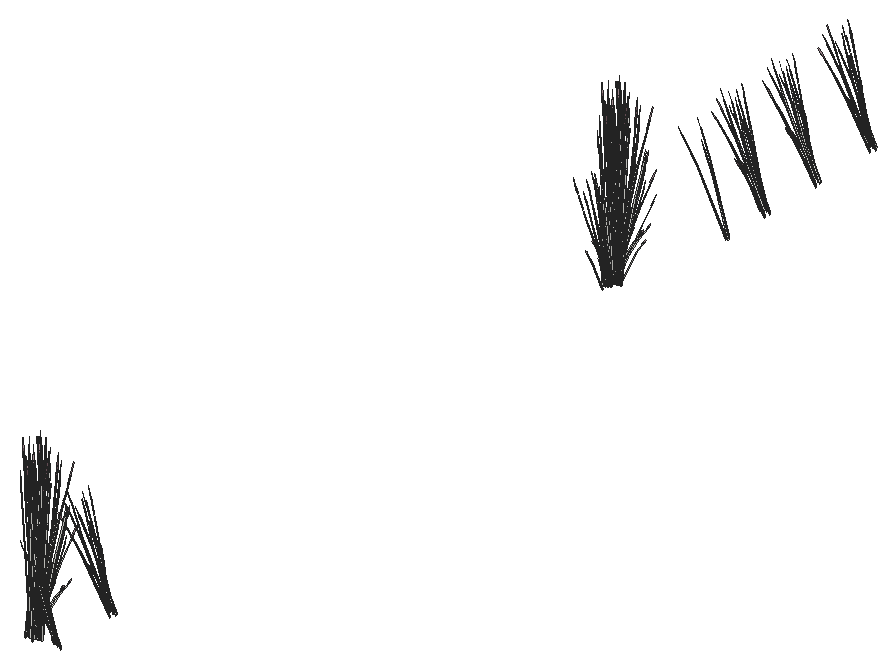
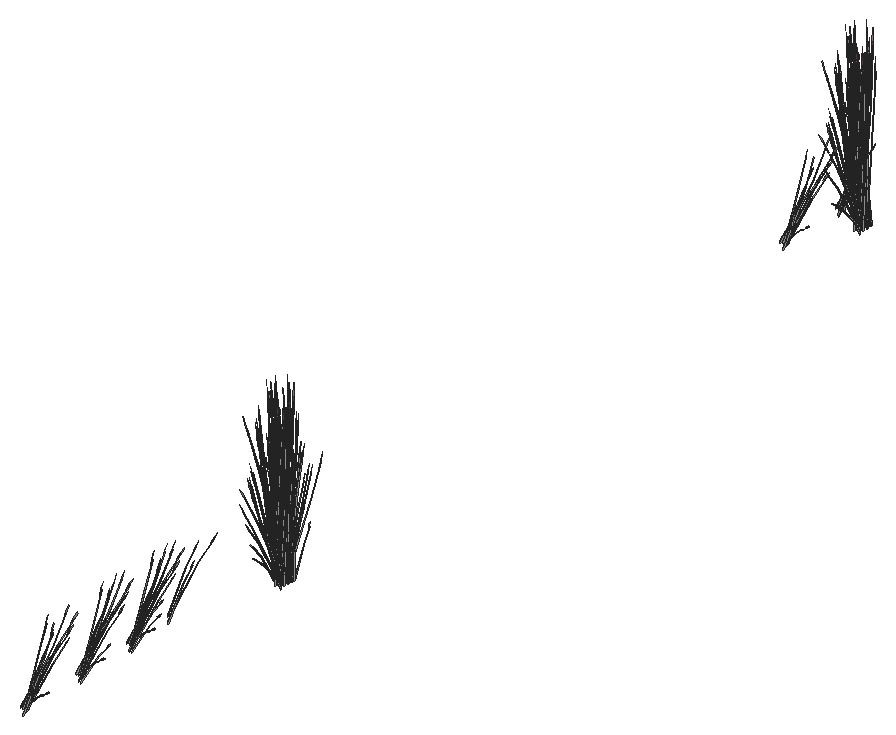
# SketchUp Ruby script. Lengths in inches.
U = 1.inch
M = Sketchup.active_model
def pt(a) = Geom::Point3d.new(a.map { |v| v * U })
def face(e, loops, mat)
  f = e.add_face(loops[0].map { |a| pt(a) })
  loops[1..].each { |l| e.add_face(l.map { |a| pt(a) }).erase! }
  f.material = f.back_material = mat if mat
  f
end
# faces: each face lists its corners as indices into pts; further lists are holes
def faces(e, pts, list, mat = nil) = list.each { |f| face(e, (f[0].is_a?(Array) ? f : [f]).map { |l| l.map { |i| pts[i] } }, mat) }
# xy, xz, yz: faces in a plane at the given z, y or x. An outline is a flat list of corners, or four numbers for a rectangle; further outlines are holes
def ring(l) = l.size == 4 ? [[l[0], l[1]], [l[2], l[1]], [l[2], l[3]], [l[0], l[3]]] : l.each_slice(2).to_a
def flat(e, list, mat, &to3) = list.each { |f| face(e, (f[0].is_a?(Array) ? f : [f]).map { |l| ring(l).map { |u, v| to3.(u, v) } }, mat) }
def xy(e, z, list, mat = nil) = flat(e, list, mat) { |x, y| [x, y, z] }
def xz(e, y, list, mat = nil) = flat(e, list, mat) { |x, z| [x, y, z] }
def yz(e, x, list, mat = nil) = flat(e, list, mat) { |y, z| [x, y, z] }
def lines(e, pts, list) = list.each { |a, b| e.add_line(pt(pts[a]), pt(pts[b])) }
# prism: a flat outline (further loops are holes) pulled along v
def prism(e, loops, v, mat = nil)
  f = face(e, loops, mat); d = Geom::Vector3d.new(v.map { |x| x * U })
  f.pushpull(f.normal.samedirection?(d) ? d.length : -d.length)
end
def box(e, o, s, mat = nil) = prism(e, [[o, [o[0] + s[0], o[1], o[2]], [o[0] + s[0], o[1] + s[1], o[2]], [o[0], o[1] + s[1], o[2]]]], [0, 0, s[2]], mat)
def at(x, y, z, deg = 0) = Geom::Transformation.translation(pt([x, y, z])) * Geom::Transformation.rotation(ORIGIN, Z_AXIS, deg.degrees)
def axes(o, x, y, z) = Geom::Transformation.new([*x, 0, *y, 0, *z, 0, *pt(o).to_a, 1])
def part(name) = M.definitions.add(name)
# library, detail: a bought-in or finely detailed component or shape, given as its bounding box
def library(name, o, s) = part(name).tap { |d| box(d.entities, o, s) }
def detail(e, o, s) = box(e.add_group.entities, o, s)
def put(e, d, t, mat = nil) = e.add_instance(d, t).tap { |i| i.material = mat if mat }
def group(e, t, mat = nil) = e.add_group.tap { |g| g.transformation = t; g.material = mat if mat }.entities
root = M.entities
M.materials.add("LightPink_Translucent").color = [144, 107, 117]
M.materials["LightPink_Translucent"].alpha = 0.75
c1 = part("blade")
p = [[2.15,0.21,22],[0,0.17,0],[0.09,0.45,0],[2.18,0.31,22],[2.29,0.31,22],[0.38,0.45,0],
  [2.48,0.24,33],[2.49,0.24,33],[2.48,0.22,33]]
faces(c1.entities,p,[[0,1,2,3],[4,5,2,3],[6,3,4,7],[8,0,3,6]])
c2 = part("seeds")
p = [[0.3,-0.1,1.38],[-0.01,-0.03,1.59],[-0.01,-0.03,0.03],[0.14,-0.07,-0.07],[0.29,-0.03,3],[0.15,0.01,3.11]]
faces(c2.entities,p,[[0,1,2,3],[1,0,4,5]],"LightPink_Translucent")
c3 = part("blade with seeds")
put(c3.entities,c1,at(0,0,0))
put(c3.entities,c2,axes([2.4,0.25,30.99],[1.5799,-0.05474,1.17369],[-0.12525,1.92788,0.29478],[-0.07173,-0.02425,1.56792]))
put(root,c3,axes([492.53,187.29,1.91],[-0.82508,0.03772,0.44739],[-0.07462,-0.62614,-0.21531],[0.14771,-0.06346,1.43643]))
put(root,c3,axes([492.5,187.51,1.55],[0.33034,0.68327,0.45755],[-0.94388,0.2376,0.17955],[0.01154,-0.12555,1.58856]))
put(root,c3,axes([502.6,185.86,3.72],[-0.63144,-0.17046,-0.35414],[0.18417,-0.49731,0.4572],[-0.25423,0.0456,0.87481]))
put(root,c3,axes([492.33,188.05,1.91],[-0.36864,0.55059,0.44739],[-0.76598,-0.26498,-0.21531],[0,-0.12692,1.43643]))
put(root,c3,axes([493.6875,187.57,1.4],[0,-0.70701,0],[0.95008,0,0],[0,0,1.79456]))
put(root,c3,axes([494.84,185.9375,1.67],[-0.7111,-0.30552,0.49651],[0.42504,-0.54784,0],[0.16196,0.06958,1.57504]))
put(root,c3,axes([493.24,187.125,1.55],[-0.62999,0.55453,0.45755],[-0.74845,-0.4895,0.17955],[0.15188,-0.05534,1.58856]))
put(root,c3,axes([493.92,188.12,1.49],[-0.70674,-0.52593,-0.06131],[0.70717,-0.52625,0],[-0.02468,-0.01837,1.75571]))
put(root,c3,axes([492.14,186.21,1.67],[-0.21949,0.60727,0.17642],[-0.8032,-0.17185,0.35086],[0.13875,-0.00296,1.60407]))
put(root,c3,axes([493.82,186.89,1.81],[0.14658,-0.54532,0.1448],[0.71613,0.09466,-0.41347],[0.13033,0.05599,1.26744]))
put(root,c3,axes([504.52,185.78,2.53],[0.21597,-0.08839,1.77064],[0.07448,0.61717,0.13857],[-0.4678,0.08189,0.63284]))
put(root,c3,axes([493.51,187.03,1.91],[-0.45644,-0.51287,0.44739],[0.69137,-0.36116,-0.21531],[0.14771,0.06346,1.43643]))
put(root,c3,axes([492.07,189.34,1.67],[0.81646,-0.16218,0.17642],[0.20161,0.60355,0.35086],[-0.07282,-0.08794,1.60407]))
put(root,c3,axes([502.2,186.1875,3.91],[-0.12407,0.07933,1.74944],[0.01055,0.57963,-0.27667],[-0.2844,0.07538,0.14031]))
put(root,c3,axes([503.03,186.11,3.875],[-0.20584,0.55581,-0.51099],[-0.70573,-0.19051,-0.3958],[-0.28414,0.05097,0.97773]))
put(root,c3,axes([494.33,187.73,1.4],[0.85008,0,0],[0,0.63259,0],[0,0,1.78407]))
put(root,c3,axes([494.57,186.24,1.67],[-0.81646,0.16218,0.17642],[-0.20161,-0.60355,0.35086],[0.07282,0.08794,1.60407]))
put(root,c3,axes([494.06,187.41,1.57],[-0.96033,-0.12874,0.49198],[0.19544,-0.7271,0.19306],[0.14034,0.07021,1.70813]))
put(root,c3,axes([493.29,189.2,1.4],[-0.24791,-0.5268,0],[0.70791,-0.18448,0],[0,0,1.54371]))
put(root,c3,axes([494.22,189.13,1.38],[0.79769,-0.20732,-0.19198],[0.2803,0.59721,0.00008],[0.08805,-0.02292,1.73897]))
put(root,c3,axes([494.49,189.375,1.67],[0.21949,-0.60727,0.17642],[0.8032,0.17185,0.35086],[-0.13875,0.00296,1.60407]))
put(root,c3,axes([494.3125,188,1.41],[0.53038,0.39469,0],[-0.53038,0.39469,0],[0,0,1.69266]))
put(root,c3,axes([495.75,187.83,1.67],[-0.59697,-0.44509,0.17642],[0.60159,-0.4317,0.35086],[-0.06593,0.0909,1.60407]))
put(root,c3,axes([503,186.4,3.07],[0.26363,-0.12925,1.71376],[0.22195,0.59723,0.13857],[-0.41388,0.13498,0.73262]))
put(root,c3,axes([493.12,189.44,1.39],[-0.76598,-0.27433,0],[0.36864,-0.57001,0],[0,0,1.62707]))
put(root,c3,axes([494.31,187.54,1.91],[0.36864,-0.55059,0.44739],[0.76598,0.26498,-0.21531],[0,0.12692,1.43643]))
put(root,c3,axes([494.16,187.85,1.48],[0,0.70667,-0.05637],[-0.95008,0,0],[0,0.02221,1.79368]))
put(root,c3,axes([494.23,187.35,1.4],[0.45644,0.51287,-0.44739],[-0.69137,0.36116,0.21531],[0.14771,0.06346,1.43643]))
put(root,c3,axes([502.18,187.42,1.78],[0.26405,0.05016,1.43002],[0.17019,0.51235,-0.30754],[-0.35868,0.0959,0.61141]))
put(root,c3,axes([500.82,186.78,3.9],[0.09697,0.01639,1.77383],[0.29997,0.53988,-0.16761],[-0.1985,0.1417,0.31391]))
put(root,c3,axes([496.24,187.84,1.67],[0,-0.61104,0.49651],[0.85008,0,0],[0,0.13917,1.57504]))
put(root,c3,axes([494.11,188.3,1.91],[0.82508,-0.03772,0.44739],[0.07462,0.62614,-0.21531],[-0.14771,0.06346,1.43643]))
put(root,c3,axes([494.625,187.66,1.81],[0.70791,-0.1782,0.1448],[0.24791,0.50885,-0.41347],[0,0.11199,1.26744]))
put(root,c3,axes([493.99,189.45,1.4],[0.76598,0.27433,0],[-0.36864,0.57001,0],[0,0,1.74954]))
put(root,c3,axes([494.125,188.57,1.81],[0.56134,0.36712,0.1448],[-0.46823,0.41419,-0.41347],[-0.13033,0.05599,1.26744]))
put(root,c3,axes([494.72,189.7,1.67],[0.7111,-0.30552,0.49651],[0.42504,0.54784,0],[-0.16196,0.06958,1.57504]))
put(root,c3,axes([493.71,189.22,1.48],[0.33034,0.70197,-0.06012],[-0.94388,0.24598,0],[0.01154,0.02451,1.72173]))
put(root,c3,axes([496.4375,188.3,1.39],[-0.94962,-0.00489,-0.04976],[0,-0.68292,0.49943],[-0.02984,0.15546,1.58352]))
put(root,c3,axes([494.38,187.7,1.86],[0.85568,0.29155,-0.29095],[-0.41201,0.61537,-0.50002],[0.02689,0.15109,1.59708]))
put(root,c3,axes([496.24,188.4,1.22],[-0.53038,0.38124,-0.30978],[-0.53038,-0.38124,0.30978],[0,0.1228,1.38974]))
put(root,c3,axes([494.29,188.16,1.4],[-0.36864,0.55059,-0.44739],[-0.76598,-0.26498,0.21531],[0,0.12692,1.43643]))
put(root,c3,axes([494.08,189.93,4.24],[-0.11735,-0.49217,0.35414],[0.67083,-0.12996,-0.4572],[0.18018,0.14104,0.87481]))
put(root,c3,axes([494.3125,189.74,1.52],[0.95122,0.19861,0.30756],[-0.23797,0.7099,-0.36492],[-0.15744,0.08885,1.64885]))
put(root,c3,axes([496.6,188.41,1.21],[0,0.61104,-0.49651],[-0.85008,0,0],[0,0.13917,1.57504]))
put(root,c3,axes([494.53,187.09,3.67],[-0.65655,-0.31748,1.38283],[0.69326,-0.49431,0.59665],[0.21183,0.29789,1.33663]))
put(root,c3,axes([494.89,190.125,1.57],[0.47504,0.61229,0],[-0.79476,0.34146,-0.51607],[-0.18101,0.07777,1.63711]))
put(root,c3,axes([493.43,190.61,3.9],[0.00225,-0.07398,1.77383],[0.65113,-0.32638,-0.16761],[0.22617,0.1165,0.31391]))
put(root,c3,axes([494.72,188.33,1.29],[0.2786,0.55945,-0.69212],[-0.80253,0.20149,-0.18165],[0.03079,0.18945,1.52773]))
put(root,c3,axes([492.48,190,4.24],[0.22906,-0.4699,0.35414],[0.66828,0.13705,-0.4572],[0.06128,0.18919,0.87481]))
put(root,c3,axes([494.19,190.37,3.92],[-0.34533,0.38816,0.0643],[-0.49176,-0.22599,0.50621],[0.15898,0.12445,0.77189]))
put(root,c3,axes([493.38,191.68,4.84],[0.52505,-0.35054,-0.06488],[0.48109,0.38392,-0.29416],[0.03387,0.10878,0.97024]))
put(root,c3,axes([494.33,190.26,3.93],[-0.75571,0.14023,0.48003],[-0.13115,-0.55007,0.3958],[0.17773,0.16212,0.9933]))
put(root,c3,axes([492.27,190.43,3.92],[-0.55987,0.20767,0.0643],[-0.27403,-0.37869,0.50621],[0.05407,0.16693,0.77189]))
put(root,c3,axes([492.26,190.2,4.23],[0.74352,-0.28449,-0.1216],[0.36538,0.50492,-0.67495],[0.0981,0.21277,1.02557]))
put(root,c3,axes([492.47,190.39,4.26],[-0.74868,-0.15974,0.53283],[0.25601,-0.52518,0.43934],[0.04499,0.20653,1.10256]))
put(root,c3,axes([492.39,190.3125,0.6875],[0.12297,-0.03325,1.76342],[0.73967,0.18301,-0.26939],[0.02163,0.20626,0.30037]))
put(root,c3,axes([492.89,190.18,3.875],[0.7469,0.15318,-0.51099],[-0.25601,0.52518,-0.3958],[0.06849,0.21144,0.97773]))
put(root,c3,axes([493.32,189.09,3.07],[-0.17368,-0.19618,1.71376],[0.80256,-0.16516,0.13857],[0.18139,0.30799,0.73262]))
put(root,c3,axes([492.55,190.5,3.72],[-0.22906,0.4699,-0.35414],[-0.66828,-0.13705,0.4572],[0.06128,0.18919,0.87481]))
put(root,c3,axes([492.62,190.08,4.17],[0.36264,0.49684,-0.71045],[-0.74649,0.27689,0.08574],[0.0848,0.24006,1.00501]))
put(root,c3,axes([492.08,191.33,3.91],[0.09631,0.0984,1.74944],[0.77725,0.03866,-0.27667],[0.07816,0.217,0.14031]))
put(root,c3,axes([503.6,208.63,3.07],[0.28223,0.10528,1.71376],[-0.58406,0.44165,0.13857],[-0.36402,-0.19924,0.73262]))
put(root,c3,axes([503.33,209.1875,1.78],[0.14835,0.17012,1.43002],[-0.34183,0.46242,-0.30754],[-0.351,-0.11053,0.61141]))
put(root,c3,axes([503.95,209.04,4.17],[-0.75952,-0.01471,-0.71045],[0.05101,-0.61953,0.08574],[-0.32177,-0.06538,1.00501]))
put(root,c3,axes([503,209.6,3.07],[0.31515,-0.01384,1.71376],[-0.20907,0.5998,0.13857],[-0.44912,-0.0371,0.73262]))
put(root,c3,axes([502.73,210.11,3.72],[-0.63144,-0.17046,-0.35414],[0.18417,-0.49731,0.4572],[-0.25423,0.0456,0.87481]))
put(root,c3,axes([504.65,210.03,2.53],[0.21597,-0.08839,1.77064],[0.07448,0.61717,0.13857],[-0.4678,0.08189,0.63284]))
put(root,c3,axes([502.33,210.44,3.91],[-0.12407,0.07933,1.74944],[0.01055,0.57963,-0.27667],[-0.2844,0.07538,0.14031]))
put(root,c3,axes([503.16,210.36,3.875],[-0.20584,0.55581,-0.51099],[-0.70573,-0.19051,-0.3958],[-0.28414,0.05097,0.97773]))
put(root,c3,axes([503.14,210.65,3.07],[0.26363,-0.12925,1.71376],[0.22195,0.59723,0.13857],[-0.41388,0.13498,0.73262]))
put(root,c3,axes([502.3125,211.67,1.78],[0.26405,0.05016,1.43002],[0.17019,0.51235,-0.30754],[-0.35868,0.0959,0.61141]))
put(root,c3,axes([500.95,211.03,3.9],[0.09697,0.01639,1.77383],[0.29997,0.53988,-0.16761],[-0.1985,0.1417,0.31391]))
put(root,c3,axes([494.39,440.3,1.78],[-0.21597,0.12368,1.43002],[-0.64681,-0.21647,-0.30754],[0.1199,-0.26922,0.61141]))
put(root,c3,axes([493.4,440.73,4.17],[-0.36264,-0.49684,-0.71045],[0.74649,-0.27689,0.08574],[-0.0848,-0.24006,1.00501]))
put(root,c3,axes([492.78,439.625,0.6875],[-0.12744,0.02202,1.76342],[-0.70477,-0.24781,-0.26939],[0.01183,-0.2067,0.30037]))
put(root,c3,axes([494.91,441.21,4.17],[0.01977,-0.56521,-0.71045],[0.83252,0.03796,0.08574],[0.08786,-0.23945,1.00501]))
put(root,c3,axes([496.07,440.33,3.91],[-0.00733,-0.12161,1.74944],[-0.61946,-0.35147,-0.27667],[0.09577,-0.21306,0.14031]))
put(root,c3,axes([493.47,440.31,3.72],[0.22906,-0.4699,-0.35414],[0.66828,0.13705,0.4572],[-0.06128,-0.18919,0.87481]))
put(root,c3,axes([495.91,439.89,3.9],[-0.07716,0.04667,1.77383],[-0.75601,-0.15746,-0.16761],[-0.02737,-0.20368,0.31391]))
put(root,c3,axes([493.59,439.3125,1.96],[0.09747,0.35631,1.1486],[-0.54071,-0.19735,0.84392],[0.05818,-0.18244,0.25299]))
put(root,c3,axes([494.74,441.03,3.875],[-0.54391,-0.41056,-0.51099],[0.57458,-0.35956,-0.3958],[0.08276,-0.2086,0.97773]))
put(root,c3,axes([493.55,440.41,3.93],[0.74868,0.15974,0.48003],[-0.25601,0.52518,0.3958],[-0.04499,-0.20653,0.9933]))
put(root,c3,axes([495.3125,441.24,4.23],[-0.83505,-0.03027,-0.1216],[0.02282,-0.57322,-0.67495],[0.05801,-0.22077,1.02557]))
put(root,c3,axes([495.26,440.875,3.72],[0.5141,-0.32171,-0.35414],[0.48666,0.36734,0.4572],[0.07405,-0.18664,0.87481]))
put(root,c3,axes([493.75,440.375,3.92],[0.55987,-0.20767,0.0643],[0.27403,0.37869,0.50621],[-0.05407,-0.16693,0.77189]))
put(root,c3,axes([493.54,440.8,4.24],[-0.22906,0.4699,0.35414],[-0.66828,-0.13705,-0.4572],[-0.06128,-0.18919,0.87481]))
put(root,c3,axes([495.45,441.04,3.92],[0.62439,0.02847,0.0643],[-0.01712,0.42991,0.50621],[0.06534,-0.16468,0.77189]))
put(root,c3,axes([494.99,441.33,4.24],[-0.5141,0.32171,0.35414],[-0.48666,-0.36734,-0.4572],[0.07405,-0.18664,0.87481]))
put(root,c3,axes([491.6,440.79,1.57],[-0.47504,-0.61229,0],[0.79476,-0.34146,-0.51607],[0.18101,-0.07777,1.63711]))
put(root,c3,axes([492.25,440.7,1.21],[0.7111,-0.30552,-0.49651],[0.42504,0.54784,0],[0.16196,-0.06958,1.57504]))
put(root,c3,axes([493.09,441.95,1.25],[0.51177,-0.45928,-0.62353],[0.63575,0.41646,-0.16365],[0.20507,-0.11457,1.37633]))
put(root,c3,axes([492.2,442.76,1.4],[0.36864,-0.55059,-0.44739],[0.76598,0.26498,0.21531],[0,-0.12692,1.43643]))
put(root,c3,axes([492.54,442.48,1.86],[-0.08854,-0.69723,-0.29095],[0.92215,-0.04216,-0.50002],[0.16238,-0.09287,1.59708]))
put(root,c3,axes([492.41,440.9375,1.22],[0.70886,0.15119,-0.30978],[-0.17848,0.53243,0.30978],[0.1429,-0.0614,1.38974]))
put(root,c3,axes([492.66,443.03,1.625],[0.8561,0.29616,0.24065],[-0.41201,0.61537,0.50002],[0,-0.14185,1.60543]))
put(root,c3,axes([492.38,442.62,1.91],[-0.82508,0.03772,0.44739],[-0.07462,-0.62614,-0.21531],[0.14771,-0.06346,1.43643]))
put(root,c3,axes([492.35,442.84,1.55],[0.33034,0.68327,0.45755],[-0.94388,0.2376,0.17955],[0.01154,-0.12555,1.58856]))
put(root,c3,axes([492.1875,443.38,1.91],[-0.36864,0.55059,0.44739],[-0.76598,-0.26498,-0.21531],[0,-0.12692,1.43643]))
put(root,c3,axes([493.54,442.9,1.4],[0,-0.70701,0],[0.95008,0,0],[0,0,1.79456]))
put(root,c3,axes([494.69,441.27,1.67],[-0.7111,-0.30552,0.49651],[0.42504,-0.54784,0],[0.16196,0.06958,1.57504]))
put(root,c3,axes([493.09,442.45,1.55],[-0.62999,0.55453,0.45755],[-0.74845,-0.4895,0.17955],[0.15188,-0.05534,1.58856]))
put(root,c3,axes([493.78,443.45,1.49],[-0.70674,-0.52593,-0.06131],[0.70717,-0.52625,0],[-0.02468,-0.01837,1.75571]))
put(root,c3,axes([492,441.54,1.67],[-0.21949,0.60727,0.17642],[-0.8032,-0.17185,0.35086],[0.13875,-0.00296,1.60407]))
put(root,c3,axes([493.67,442.22,1.81],[0.14658,-0.54532,0.1448],[0.71613,0.09466,-0.41347],[0.13033,0.05599,1.26744]))
put(root,c3,axes([493.37,442.36,1.91],[-0.45644,-0.51287,0.44739],[0.69137,-0.36116,-0.21531],[0.14771,0.06346,1.43643]))
put(root,c3,axes([491.92,444.67,1.67],[0.81646,-0.16218,0.17642],[0.20161,0.60355,0.35086],[-0.07282,-0.08794,1.60407]))
put(root,c3,axes([494.18,443.06,1.4],[0.85008,0,0],[0,0.63259,0],[0,0,1.78407]))
put(root,c3,axes([494.43,441.57,1.67],[-0.81646,0.16218,0.17642],[-0.20161,-0.60355,0.35086],[0.07282,0.08794,1.60407]))
put(root,c3,axes([493.91,442.74,1.57],[-0.96033,-0.12874,0.49198],[0.19544,-0.7271,0.19306],[0.14034,0.07021,1.70813]))
put(root,c3,axes([493.14,444.53,1.4],[-0.24791,-0.5268,0],[0.70791,-0.18448,0],[0,0,1.54371]))
put(root,c3,axes([494.07,444.46,1.38],[0.79769,-0.20732,-0.19198],[0.2803,0.59721,0.00008],[0.08805,-0.02292,1.73897]))
put(root,c3,axes([494.35,444.71,1.67],[0.21949,-0.60727,0.17642],[0.8032,0.17185,0.35086],[-0.13875,0.00296,1.60407]))
put(root,c3,axes([494.17,443.33,1.41],[0.53038,0.39469,0],[-0.53038,0.39469,0],[0,0,1.69266]))
put(root,c3,axes([495.6,443.16,1.67],[-0.59697,-0.44509,0.17642],[0.60159,-0.4317,0.35086],[-0.06593,0.0909,1.60407]))
put(root,c3,axes([492.97,444.77,1.39],[-0.76598,-0.27433,0],[0.36864,-0.57001,0],[0,0,1.62707]))
put(root,c3,axes([494.16,442.87,1.91],[0.36864,-0.55059,0.44739],[0.76598,0.26498,-0.21531],[0,0.12692,1.43643]))
put(root,c3,axes([494.02,443.18,1.48],[0,0.70667,-0.05637],[-0.95008,0,0],[0,0.02221,1.79368]))
put(root,c3,axes([494.09,442.68,1.4],[0.45644,0.51287,-0.44739],[-0.69137,0.36116,0.21531],[0.14771,0.06346,1.43643]))
put(root,c3,axes([496.09,443.17,1.67],[0,-0.61104,0.49651],[0.85008,0,0],[0,0.13917,1.57504]))
put(root,c3,axes([493.96,443.63,1.91],[0.82508,-0.03772,0.44739],[0.07462,0.62614,-0.21531],[-0.14771,0.06346,1.43643]))
put(root,c3,axes([494.48,442.99,1.81],[0.70791,-0.1782,0.1448],[0.24791,0.50885,-0.41347],[0,0.11199,1.26744]))
put(root,c3,axes([493.84,444.78,1.4],[0.76598,0.27433,0],[-0.36864,0.57001,0],[0,0,1.74954]))
put(root,c3,axes([493.98,443.9,1.81],[0.56134,0.36712,0.1448],[-0.46823,0.41419,-0.41347],[-0.13033,0.05599,1.26744]))
put(root,c3,axes([494.57,445.03,1.67],[0.7111,-0.30552,0.49651],[0.42504,0.54784,0],[-0.16196,0.06958,1.57504]))
put(root,c3,axes([493.5625,444.55,1.48],[0.33034,0.70197,-0.06012],[-0.94388,0.24598,0],[0.01154,0.02451,1.72173]))
put(root,c3,axes([496.29,443.63,1.39],[-0.94962,-0.00489,-0.04976],[0,-0.68292,0.49943],[-0.02984,0.15546,1.58352]))
put(root,c3,axes([494.24,443.03,1.86],[0.85568,0.29155,-0.29095],[-0.41201,0.61537,-0.50002],[0.02689,0.15109,1.59708]))
put(root,c3,axes([496.09,443.73,1.22],[-0.53038,0.38124,-0.30978],[-0.53038,-0.38124,0.30978],[0,0.1228,1.38974]))
put(root,c3,axes([494.14,443.49,1.4],[-0.36864,0.55059,-0.44739],[-0.76598,-0.26498,0.21531],[0,0.12692,1.43643]))
put(root,c3,axes([493.9375,445.26,4.24],[-0.11735,-0.49217,0.35414],[0.67083,-0.12996,-0.4572],[0.18018,0.14104,0.87481]))
put(root,c3,axes([494.16,445.07,1.52],[0.95122,0.19861,0.30756],[-0.23797,0.7099,-0.36492],[-0.15744,0.08885,1.64885]))
put(root,c3,axes([496.46,443.74,1.21],[0,0.61104,-0.49651],[-0.85008,0,0],[0,0.13917,1.57504]))
put(root,c3,axes([494.39,442.42,3.67],[-0.65655,-0.31748,1.38283],[0.69326,-0.49431,0.59665],[0.21183,0.29789,1.33663]))
put(root,c3,axes([495.38,445.01,1.96],[-0.4278,-0.1757,1.1486],[0.5524,-0.17852,0.84392],[0.14899,0.15122,0.25299]))
put(root,c3,axes([494.74,445.46,1.57],[0.47504,0.61229,0],[-0.79476,0.34146,-0.51607],[-0.18101,0.07777,1.63711]))
put(root,c3,axes([493.28,445.94,3.9],[0.00225,-0.07398,1.77383],[0.65113,-0.32638,-0.16761],[0.22617,0.1165,0.31391]))
put(root,c3,axes([494.58,443.66,1.29],[0.2786,0.55945,-0.69212],[-0.80253,0.20149,-0.18165],[0.03079,0.18945,1.52773]))
put(root,c3,axes([492.33,445.33,4.24],[0.22906,-0.4699,0.35414],[0.66828,0.13705,-0.4572],[0.06128,0.18919,0.87481]))
put(root,c3,axes([494.04,445.7,3.92],[-0.34533,0.38816,0.0643],[-0.49176,-0.22599,0.50621],[0.15898,0.12445,0.77189]))
put(root,c3,axes([493.23,447.01,4.84],[0.52505,-0.35054,-0.06488],[0.48109,0.38392,-0.29416],[0.03387,0.10878,0.97024]))
put(root,c3,axes([494.1875,445.59,3.93],[-0.75571,0.14023,0.48003],[-0.13115,-0.55007,0.3958],[0.17773,0.16212,0.9933]))
put(root,c3,axes([493.86,444.82,1.78],[0.01341,-0.20255,1.43002],[0.64074,-0.22625,-0.30754],[0.1978,0.24243,0.61141]))
put(root,c3,axes([492.125,445.76,3.92],[-0.55987,0.20767,0.0643],[-0.27403,-0.37869,0.50621],[0.05407,0.16693,0.77189]))
put(root,c3,axes([492.11,445.53,4.23],[0.74352,-0.28449,-0.1216],[0.36538,0.50492,-0.67495],[0.0981,0.21277,1.02557]))
put(root,c3,axes([492.32,445.72,4.26],[-0.74868,-0.15974,0.53283],[0.25601,-0.52518,0.43934],[0.04499,0.20653,1.10256]))
put(root,c3,axes([492.24,445.64,0.6875],[0.12297,-0.03325,1.76342],[0.73967,0.18301,-0.26939],[0.02163,0.20626,0.30037]))
put(root,c3,axes([492.75,445.51,3.875],[0.7469,0.15318,-0.51099],[-0.25601,0.52518,-0.3958],[0.06849,0.21144,0.97773]))
put(root,c3,axes([493.17,444.42,3.07],[-0.17368,-0.19618,1.71376],[0.80256,-0.16516,0.13857],[0.18139,0.30799,0.73262]))
put(root,c3,axes([492.41,445.83,3.72],[-0.22906,0.4699,-0.35414],[-0.66828,-0.13705,0.4572],[0.06128,0.18919,0.87481]))
put(root,c3,axes([492.48,445.41,4.17],[0.36264,0.49684,-0.71045],[-0.74649,0.27689,0.08574],[0.0848,0.24006,1.00501]))
put(root,c3,axes([491.93,446.66,3.91],[0.09631,0.0984,1.74944],[0.77725,0.03866,-0.27667],[0.07816,0.217,0.14031]))
put(root,c3,axes([504.28,479.18,3.07],[0.31515,-0.01384,1.71376],[-0.20907,0.5998,0.13857],[-0.44912,-0.0371,0.73262]))
put(root,c3,axes([504.41,480.23,3.07],[0.26363,-0.12925,1.71376],[0.22195,0.59723,0.13857],[-0.41388,0.13498,0.73262]))
put(root,c3,axes([503.59,481.25,1.78],[0.26405,0.05016,1.43002],[0.17019,0.51235,-0.30754],[-0.35868,0.0959,0.61141]))
put(root,c3,axes([503.24,497.13,3.07],[0.28223,0.10528,1.71376],[-0.58406,0.44165,0.13857],[-0.36402,-0.19924,0.73262]))
put(root,c3,axes([502.97,497.69,1.78],[0.14835,0.17012,1.43002],[-0.34183,0.46242,-0.30754],[-0.351,-0.11053,0.61141]))
put(root,c3,axes([503.58,497.54,4.17],[-0.75952,-0.01471,-0.71045],[0.05101,-0.61953,0.08574],[-0.32177,-0.06538,1.00501]))
put(root,c3,axes([502.55,496.53,3.9],[0.05633,0.06098,1.77383],[-0.27155,0.54815,-0.16761],[-0.27501,0.00397,0.31391]))
put(root,c3,axes([503.33,497.66,3.875],[-0.55171,0.40476,-0.51099],[-0.48318,-0.42758,-0.3958],[-0.28031,-0.06159,0.97773]))
put(root,c3,axes([502.64,498.1,3.07],[0.31515,-0.01384,1.71376],[-0.20907,0.5998,0.13857],[-0.44912,-0.0371,0.73262]))
put(root,c3,axes([502.44,498.83,0.6875],[0.01927,0.0963,1.76342],[-0.38846,0.5029,-0.26939],[-0.27592,-0.02535,0.30037]))
put(root,c3,axes([502.36,498.61,3.72],[-0.63144,-0.17046,-0.35414],[0.18417,-0.49731,0.4572],[-0.25423,0.0456,0.87481]))
put(root,c3,axes([504.29,498.53,2.53],[0.21597,-0.08839,1.77064],[0.07448,0.61717,0.13857],[-0.4678,0.08189,0.63284]))
put(root,c3,axes([501.96,498.94,3.91],[-0.12407,0.07933,1.74944],[0.01055,0.57963,-0.27667],[-0.2844,0.07538,0.14031]))
put(root,c3,axes([502.8,498.86,3.875],[-0.20584,0.55581,-0.51099],[-0.70573,-0.19051,-0.3958],[-0.28414,0.05097,0.97773]))
put(root,c3,axes([502.77,499.15,3.07],[0.26363,-0.12925,1.71376],[0.22195,0.59723,0.13857],[-0.41388,0.13498,0.73262]))
put(root,c3,axes([501.95,500.17,1.78],[0.26405,0.05016,1.43002],[0.17019,0.51235,-0.30754],[-0.35868,0.0959,0.61141]))
put(root,c3,axes([500.59,499.53,3.9],[0.09697,0.01639,1.77383],[0.29997,0.53988,-0.16761],[-0.1985,0.1417,0.31391]))
put(root,c3,axes([503.47,519.23,3.07],[0.28223,0.10528,1.71376],[-0.58406,0.44165,0.13857],[-0.36402,-0.19924,0.73262]))
put(root,c3,axes([503.2,519.79,1.78],[0.14835,0.17012,1.43002],[-0.34183,0.46242,-0.30754],[-0.351,-0.11053,0.61141]))
put(root,c3,axes([503.82,519.64,4.17],[-0.75952,-0.01471,-0.71045],[0.05101,-0.61953,0.08574],[-0.32177,-0.06538,1.00501]))
put(root,c3,axes([503.5625,519.76,3.875],[-0.55171,0.40476,-0.51099],[-0.48318,-0.42758,-0.3958],[-0.28031,-0.06159,0.97773]))
put(root,c3,axes([502.875,520.19,3.07],[0.31515,-0.01384,1.71376],[-0.20907,0.5998,0.13857],[-0.44912,-0.0371,0.73262]))
put(root,c3,axes([502.67,520.93,0.6875],[0.01927,0.0963,1.76342],[-0.38846,0.5029,-0.26939],[-0.27592,-0.02535,0.30037]))
put(root,c3,axes([502.6,520.71,3.72],[-0.63144,-0.17046,-0.35414],[0.18417,-0.49731,0.4572],[-0.25423,0.0456,0.87481]))
put(root,c3,axes([504.52,520.625,2.53],[0.21597,-0.08839,1.77064],[0.07448,0.61717,0.13857],[-0.4678,0.08189,0.63284]))
put(root,c3,axes([502.2,521.04,3.91],[-0.12407,0.07933,1.74944],[0.01055,0.57963,-0.27667],[-0.2844,0.07538,0.14031]))
put(root,c3,axes([503.03,520.96,3.875],[-0.20584,0.55581,-0.51099],[-0.70573,-0.19051,-0.3958],[-0.28414,0.05097,0.97773]))
put(root,c3,axes([503,521.25,3.07],[0.26363,-0.12925,1.71376],[0.22195,0.59723,0.13857],[-0.41388,0.13498,0.73262]))
put(root,c3,axes([502.18,522.27,1.78],[0.26405,0.05016,1.43002],[0.17019,0.51235,-0.30754],[-0.35868,0.0959,0.61141]))
put(root,c3,axes([500.82,521.625,3.9],[0.09697,0.01639,1.77383],[0.29997,0.53988,-0.16761],[-0.1985,0.1417,0.31391]))
put(root,c3,axes([503.6,543.48,3.07],[0.28223,0.10528,1.71376],[-0.58406,0.44165,0.13857],[-0.36402,-0.19924,0.73262]))
put(root,c3,axes([503.33,544.04,1.78],[0.14835,0.17012,1.43002],[-0.34183,0.46242,-0.30754],[-0.351,-0.11053,0.61141]))
put(root,c3,axes([503.95,543.89,4.17],[-0.75952,-0.01471,-0.71045],[0.05101,-0.61953,0.08574],[-0.32177,-0.06538,1.00501]))
put(root,c3,axes([503,544.45,3.07],[0.31515,-0.01384,1.71376],[-0.20907,0.5998,0.13857],[-0.44912,-0.0371,0.73262]))
put(root,c3,axes([502.73,544.96,3.72],[-0.63144,-0.17046,-0.35414],[0.18417,-0.49731,0.4572],[-0.25423,0.0456,0.87481]))
put(root,c3,axes([504.65,544.88,2.53],[0.21597,-0.08839,1.77064],[0.07448,0.61717,0.13857],[-0.4678,0.08189,0.63284]))
put(root,c3,axes([502.33,545.29,3.91],[-0.12407,0.07933,1.74944],[0.01055,0.57963,-0.27667],[-0.2844,0.07538,0.14031]))
put(root,c3,axes([503.16,545.21,3.875],[-0.20584,0.55581,-0.51099],[-0.70573,-0.19051,-0.3958],[-0.28414,0.05097,0.97773]))
put(root,c3,axes([503.14,545.5,3.07],[0.26363,-0.12925,1.71376],[0.22195,0.59723,0.13857],[-0.41388,0.13498,0.73262]))
put(root,c3,axes([502.3125,546.52,1.78],[0.26405,0.05016,1.43002],[0.17019,0.51235,-0.30754],[-0.35868,0.0959,0.61141]))
put(root,c3,axes([500.95,545.88,3.9],[0.09697,0.01639,1.77383],[0.29997,0.53988,-0.16761],[-0.1985,0.1417,0.31391]))
